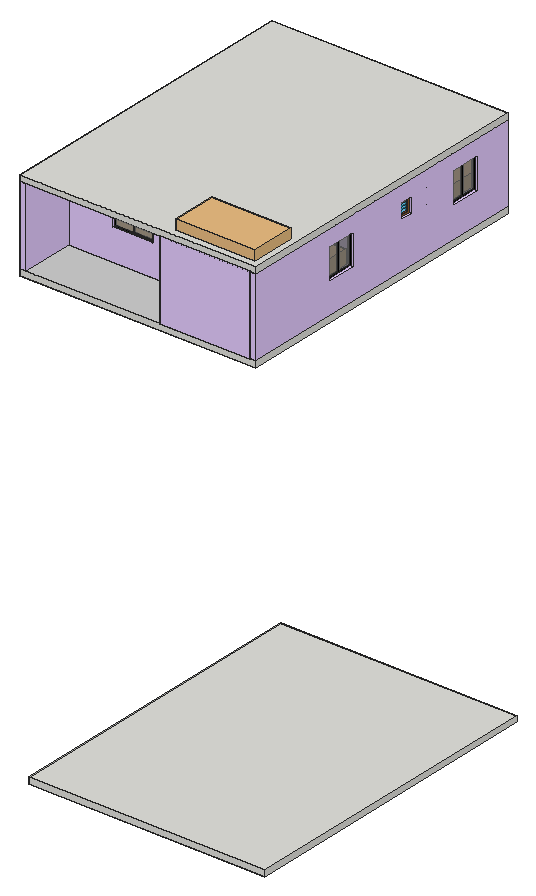
# SketchUp Ruby script. Lengths in inches.
U = 1.inch
M = Sketchup.active_model
def pt(a) = Geom::Point3d.new(a.map { |v| v * U })
def face(e, loops, mat)
  f = e.add_face(loops[0].map { |a| pt(a) })
  loops[1..].each { |l| e.add_face(l.map { |a| pt(a) }).erase! }
  f.material = f.back_material = mat if mat
  f
end
# faces: each face lists its corners as indices into pts; further lists are holes
def faces(e, pts, list, mat = nil) = list.each { |f| face(e, (f[0].is_a?(Array) ? f : [f]).map { |l| l.map { |i| pts[i] } }, mat) }
# xy, xz, yz: faces in a plane at the given z, y or x. An outline is a flat list of corners, or four numbers for a rectangle; further outlines are holes
def ring(l) = l.size == 4 ? [[l[0], l[1]], [l[2], l[1]], [l[2], l[3]], [l[0], l[3]]] : l.each_slice(2).to_a
def flat(e, list, mat, &to3) = list.each { |f| face(e, (f[0].is_a?(Array) ? f : [f]).map { |l| ring(l).map { |u, v| to3.(u, v) } }, mat) }
def xy(e, z, list, mat = nil) = flat(e, list, mat) { |x, y| [x, y, z] }
def xz(e, y, list, mat = nil) = flat(e, list, mat) { |x, z| [x, y, z] }
def yz(e, x, list, mat = nil) = flat(e, list, mat) { |y, z| [x, y, z] }
def lines(e, pts, list) = list.each { |a, b| e.add_line(pt(pts[a]), pt(pts[b])) }
# prism: a flat outline (further loops are holes) pulled along v
def prism(e, loops, v, mat = nil)
  f = face(e, loops, mat); d = Geom::Vector3d.new(v.map { |x| x * U })
  f.pushpull(f.normal.samedirection?(d) ? d.length : -d.length)
end
def box(e, o, s, mat = nil) = prism(e, [[o, [o[0] + s[0], o[1], o[2]], [o[0] + s[0], o[1] + s[1], o[2]], [o[0], o[1] + s[1], o[2]]]], [0, 0, s[2]], mat)
def at(x, y, z, deg = 0) = Geom::Transformation.translation(pt([x, y, z])) * Geom::Transformation.rotation(ORIGIN, Z_AXIS, deg.degrees)
def axes(o, x, y, z) = Geom::Transformation.new([*x, 0, *y, 0, *z, 0, *pt(o).to_a, 1])
def part(name) = M.definitions.add(name)
# library, detail: a bought-in or finely detailed component or shape, given as its bounding box
def library(name, o, s) = part(name).tap { |d| box(d.entities, o, s) }
def detail(e, o, s) = box(e.add_group.entities, o, s)
def put(e, d, t, mat = nil) = e.add_instance(d, t).tap { |i| i.material = mat if mat }
def group(e, t, mat = nil) = e.add_group.tap { |g| g.transformation = t; g.material = mat if mat }.entities
root = M.entities
M.materials.add("[0012_Bisque]").color = [255, 228, 196]
M.materials.add("[Carrera Marble]").color = [207, 207, 207]
M.materials.add("[Color A01]").color = [255, 204, 204]
M.materials.add("[Color B02]").color = [255, 178, 153]
M.materials.add("[Color B07]").color = [153, 38, 0]
M.materials.add("[Color C01]").color = [255, 229, 204]
M.materials.add("[Color C02]").color = [255, 204, 153]
M.materials.add("[Color C07]").color = [153, 76, 0]
M.materials.add("[Color J01]").color = [229, 204, 255]
M.materials.add("[Color K01]").color = [255, 204, 255]
M.materials.add("[Color M02]").color = [198, 198, 198]
M.materials.add("[Color M09]").color = [0, 0, 0]
M.materials.add("[Color_008]").color = [30, 30, 30]
M.materials.add("[Color_009]").color = [0, 0, 0]
M.materials.add("[Metal Corrugated Shiny]").color = [193, 193, 193]
M.materials.add("[Stone Marble]").color = [143, 138, 136]
M.materials.add("[Translucent Glass Gray]").color = [128, 128, 128]
M.materials["[Translucent Glass Gray]"].alpha = 0.5
M.materials.add("[Translucent Glass Tinted]1").color = [7, 201, 240]
M.materials["[Translucent Glass Tinted]1"].alpha = 0.48
M.materials.add("[Translucent_Glass_Gray]").color = [128, 128, 128]
M.materials["[Translucent_Glass_Gray]"].alpha = 0.5
M.materials.add("[Wood Cherry Original]").color = [152, 86, 42]
M.materials.add("[Wood Floor Parquet]").color = [145, 89, 39]
M.materials.add("[Wood Veneer 01]").color = [120, 70, 37]
c1 = library("main+door",[0,-0.79,0],[47.24,7.88,82.68])
c2 = library("Gas cooktop",[0,0,34.52],[24.41,48.07,2.63])
c3 = part("Inclined chimney")
g1 = group(c3.entities,at(1.97,2.08,2.89))
xy(g1,0,[[0,7.9,31.3,13.68]])
xy(g1,11.29,[[0,0,31.3,13.68]])
xz(g1,13.68,[[0,0,31.3,11.29]])
yz(g1,0,[[7.9,0,0,11.29,13.68,11.29,13.68,0]])
yz(g1,31.3,[[7.9,0,13.68,0,13.68,11.29,0,11.29]])
g2 = group(c3.entities,at(0,9.85,0.4))
g3 = group(g2,at(0,0.61,0.43))
prism(g3,[[[35.24,0,0],[35.24,-3.39,4.84],[35.24,-3.58,4.7],[35.24,-0.29,0]]],[-35.24,0,0])
g4 = group(g2,at(0,-3.21,4.99))
prism(g4,[[[35.24,-0.2,-0.12],[35.24,-3.16,5],[0,-3.16,5],[0,-0.2,-0.12]]],[0,0.2,0.12])
g5 = group(g2,at(0,-6.27,10.27))
prism(g5,[[[35.24,-0.19,-0.14],[35.24,-3.58,4.7],[0,-3.58,4.7],[0,-0.19,-0.14]]],[0,0.19,0.14])
g6 = group(g2,at(0,0.61,0.43))
prism(g6,[[[35.24,0,0],[35.24,0.96,0],[35.24,-9.52,14.96],[35.24,-10.16,14.51]]],[-35.24,0,0])
g7 = group(c3.entities,at(10.24,3.95,20.8))
box(g7,[0,0,-6.62],[14.76,11.8125,20.56])
g8 = group(c3.entities,at(0,10.1,0))
prism(g8,[[[35.24,0.46,0],[35.24,1.33,0],[35.24,1.33,0.83],[35.24,1.01,0.83],[35.24,0.37,0.83],[35.24,0,0.83],[35.24,0,0.64]]],[-35.24,0,0])
c4 = part("Inclined+chimney")
put(c4.entities,c3,at(34.17,38.97,0.69))
c5 = library("Component\#33",[0,0,0],[60.64,55.48,158.625])
c6 = library("SKT_Nearly Natural 5' Kentia Palm Silk Tree",[-23.18,-17.61,0],[47.48,43.95,59.125])
c7 = library("Bed",[-100.55,9.74,0],[90.43,103.1,58.68])
c8 = library("2222",[-1.18,-2.36,0],[94.72,146.45,38.04])
c9 = library("CS300DRT",[0,0,0],[27.18,17.85,30.31])
c10 = library("Oval wall hanging",[0,0,0],[26.88,1.18,49.49])
c11 = part("ventilator")
g9 = group(c11.entities,at(0,0,0))
xy(g9,0,[[0,0,24,1],[0,1,24,6.83]],"[Wood Floor Parquet]")
xy(g9,1.75,[[2,0,22,6.83]],"[Wood Floor Parquet]")
xy(g9,21.87,[[2,0,22,6.83]],"[Wood Cherry Original]")
xy(g9,23.62,[[0,0,24,1],[0,1,24,6.83]],"[Wood Floor Parquet]")
xz(g9,0,[[[0,0,24,23.62],[2,1.75,22,21.87]]],"[Wood Floor Parquet]")
xz(g9,6.83,[[[0,0,24,23.62],[2,1.75,22,21.87]]],"[Wood Cherry Original]")
yz(g9,0,[[0,0,1,23.62],[1,0,6.83,23.62]],"[Wood Floor Parquet]")
yz(g9,2,[[0,1.75,6.83,1.75,6.83,7.66,0,3.5],[0,3.5,6.83,7.66,6.83,11.8125,0,7.66],[0,7.66,6.83,11.8125,6.83,15.97,0,11.8125],[0,11.8125,6.83,15.97,6.83,20.12,0,15.97],[0,15.97,6.83,20.12,6.83,21.87,0,21.87]],"[Wood Floor Parquet]")
yz(g9,22,[[0,1.75,0,3.5,6.83,7.66,6.83,1.75],[0,3.5,0,7.66,6.83,11.8125,6.83,7.66],[0,7.66,0,11.8125,6.83,15.97,6.83,11.8125],[0,11.8125,0,15.97,6.83,20.12,6.83,15.97],[0,15.97,0,21.87,6.83,21.87,6.83,20.12]],"[Wood Floor Parquet]")
yz(g9,24,[[0,0,1,23.62],[1,0,6.83,23.62]],"[Wood Floor Parquet]")
p = [[2,0,3.5],[2,6.83,7.66],[22,6.83,7.66],[22,0,3.5],[2,6.83,11.8125],[2,0,7.66],
  [22,0,7.66],[22,6.83,11.8125],[2,0,11.8125],[2,6.83,15.97],[22,6.83,15.97],[22,0,11.8125],
  [2,6.83,20.12],[2,0,15.97],[22,0,15.97],[22,6.83,20.12]]
faces(g9,p,[[0,1,2,3],[4,5,6,7],[8,9,10,11]],"[Translucent Glass Tinted]1")
faces(g9,p,[[12,13,14,15]],"[Translucent Glass Gray]")
c12 = part("Group\#32")
xy(c12.entities,0,[[0,0,82.68,1.18]],"[Color_009]")
xy(c12.entities,1.97,[[1.97,0.98,40.35,1.18],[42.32,0.98,80.71,1.18]])
xy(c12.entities,1.97,[[1.97,0,40.35,0.3],[42.32,0,80.71,0.3]],"[Color_009]")
xy(c12.entities,80.71,[[1.97,0,40.35,0.3],[42.32,0,80.71,0.3],[1.97,0.3,40.35,0.98],[42.32,0.3,80.71,0.98],[1.97,0.98,40.35,1.18],
  [42.32,0.98,80.71,1.18]])
xy(c12.entities,82.68,[[0,0,82.68,1.18]],"[Color_008]")
xz(c12.entities,0,[[[0,0,82.68,82.68],[1.97,1.97,40.35,80.71],[42.32,1.97,80.71,80.71]]],"[Color_009]")
xz(c12.entities,0.3,[[1.97,1.97,40.35,80.71],[42.32,1.97,80.71,80.71]],"[Translucent_Glass_Gray]")
xz(c12.entities,0.98,[[1.97,1.97,40.35,80.71],[42.32,1.97,80.71,80.71]],"[Translucent_Glass_Gray]")
xz(c12.entities,1.18,[[[0,0,82.68,82.68],[1.97,1.97,80.71,80.71]],[40.35,1.97,42.32,80.71]],"[Color_009]")
yz(c12.entities,0,[[0,0,1.18,82.68]],"[Color_009]")
yz(c12.entities,1.97,[[0.98,1.97,1.18,80.71]])
yz(c12.entities,1.97,[[0,1.97,0.3,80.71]],"[Color_009]")
yz(c12.entities,40.35,[[0,1.97,0.3,80.71],[0.98,1.97,1.18,80.71]],"[Color_009]")
yz(c12.entities,42.32,[[0,1.97,0.3,80.71],[0.98,1.97,1.18,80.71]])
yz(c12.entities,80.71,[[0,1.97,0.3,80.71],[0.98,1.97,1.18,80.71]],"[Color_009]")
yz(c12.entities,82.68,[[0,0,1.18,82.68]],"[Color_009]")
c13 = library("Group53\#1",[561.19,10.9375,5.6875],[120.56,68.625,137.75])
c14 = part("Vertical frame member")
xy(c14.entities,-6,[[0,-2,2.13,0]])
xy(c14.entities,78,[[0,-2,2.13,0]])
xz(c14.entities,-2,[[0,-6,2.13,78]],"[Color B07]")
xz(c14.entities,0,[[0,-6,2.13,78]])
yz(c14.entities,0,[[-2,-6,0,78]])
yz(c14.entities,2.13,[[-2,-6,0,78]])
c15 = part("Group\#9")
p = [[2,2,2],[2,2,4],[2,-0.06,4]]
lines(c15.entities,p,[[0,1],[1,2]])
g10 = group(c15.entities,at(0,0,0))
xy(g10,2,[[2,0,8,2]])
xy(g10,4,[[0,0,8,2]])
xz(g10,0,[[0,0,2,0,2,2,8,2,8,4,0,4]])
xz(g10,2,[[0,0,0,4,8,4,8,2,2,2,2,0]])
yz(g10,0,[[0,0,2,4]])
yz(g10,2,[[0,0,2,2]])
yz(g10,8,[[0,2,2,4]])
g11 = group(c15.entities,at(8,0,0))
xy(g11,4,[[0,0,2,2]])
xz(g11,0,[[0,0,2,4]])
xz(g11,2,[[0,0,2,4]])
yz(g11,0,[[0,0,2,4]])
yz(g11,2,[[0,0,2,4]])
c16 = part("Cabinet pull")
p = [[1,1,1],[2,1,1],[2,1,0]]
lines(c16.entities,p,[[0,1],[1,2]])
g12 = group(c16.entities,at(0,8,0),"[Metal Corrugated Shiny]")
xy(g12,0,[[0,0,2,1]])
xy(g12,1,[[0,0,2,1]])
xz(g12,0,[[0,0,2,1]])
xz(g12,1,[[0,0,1,1],[1,0,2,1]])
yz(g12,2,[[0,0,1,1]])
g13 = group(c16.entities,at(0,0,0),"[Metal Corrugated Shiny]")
xy(g13,0,[[0,0,0,1,1,1,1,8,2,8,2,0]])
xy(g13,1,[[0,0,2,0,2,8,1,8,1,1,0,1]])
xz(g13,0,[[0,0,2,1]])
xz(g13,1,[[0,0,1,1]])
xz(g13,8,[[1,0,2,1]])
yz(g13,1,[[1,0,8,1]])
yz(g13,2,[[0,0,8,1]])
c17 = part("Rectangular panel")
box(c17.entities,[0,0,0],[0.4375,33.64,17.64])
c18 = part("Group\#14")
xy(c18.entities,18.12,[[0,0,28.25,0.25]])
xz(c18.entities,0,[[0,0,28.25,18.12]])
yz(c18.entities,0,[[0,0.43,0.25,18.12]])
yz(c18.entities,28.25,[[0,0.43,0.25,17.43],[0,17.43,0.25,18.12]])
xy(root,0,[[228.5,1157.72,238.5,1187.97],[238.5,1157.72,248.5,1187.97],[248.5,1157.72,258.5,1187.97],[258.5,1157.72,268.5,1187.97],[268.5,1157.72,278.5,1187.97],
  [278.5,1157.72,288.5,1187.97],[288.5,1157.72,298.5,1187.97],[298.5,1157.72,308.5,1187.97],[308.5,1157.72,318.5,1187.97],[318.5,1157.72,351,1187.97],
  [318.5,1187.97,351,1199.97],[228.5,1199.97,238.5,1230.22],[238.5,1199.97,248.5,1230.22],[248.5,1199.97,258.5,1230.22],[258.5,1199.97,268.5,1230.22],
  [268.5,1199.97,278.5,1230.22],[278.5,1199.97,288.5,1230.22],[288.5,1199.97,298.5,1230.22],[298.5,1199.97,308.5,1230.22],[308.5,1199.97,318.5,1230.22],
  [318.5,1199.97,351,1230.22]])
p = [[-296.69,1230.22,0],[-295.69,1230.22,0],[-296.69,1235.22,0],[-332.69,1230.22,0],[-332.69,1235.22,0],[-295.69,1266.22,0],
  [-296.69,1266.22,0],[81.8,1619.72,48],[81.8,1619.72,96],[33.8,1619.72,96],[33.8,1619.72,48],[212.75,1235.22,0],
  [9,1235.22,0],[9,1541.6,0],[212.75,1541.6,0],[213.32,1157.72,120],[213.32,1230.22,120]]
lines(root,p,[[0,1],[0,2],[3,4],[5,6],[7,8],[8,9],[9,10],[10,7],[11,12],[12,13],[14,11],[15,16]])
put(root,c1,axes([261.5,1465.22,0],[0,-0.762,0],[0.735,0,0],[0,0,1.016]))
put(root,c2,at(9.27,1518.85,9.47))
put(root,c4,axes([63.73,1499.16,69.82],[0,0.81,0],[-1,0,0],[0,0,0.88]))
put(root,c5,axes([35.81,1464.81,0],[0,0.46858,0],[-0.5529,0,0],[0,0,0.52253]))
put(root,c6,axes([24.22,1605.45,43.99],[0.68,0,0],[0,0.68,0],[0,0,0.5236]))
put(root,c7,axes([226.75,1495.01,0],[0,-1.24,0],[1,0,0],[0,0,1]))
put(root,c7,axes([348.23,1359.9,0],[0,1.24,0],[-1,0,0],[0,0,1]))
put(root,c8,at(29.45,1246.26,0))
put(root,c9,axes([134.5,1569.67,0],[1.5,0,0],[0,1.5,0],[0,0,1.5]))
put(root,c10,axes([162.44,1617.36,58.25],[1,0,0],[0,2,0],[0,0,1]))
put(root,c9,axes([351,1451.89,0],[-1.5,0,0],[0,-1.5,0],[0,0,1.5]))
g14 = group(root,at(0,1148.64,0),"[Color J01]")
xy(g14,0,[[213.32,0,213.32,9.09,351,9.09,351,81.59,208.5,81.59,208.5,86.59,213.5,86.59,213.5,242.59,223.5,242.59,223.5,237.59,218.5,237.59,218.5,86.59,351,86.59,351,186.09,360,186.09,360,0.09,351,0.09,351,0],[0,0.09,0,122.64,9,122.64,9,86.59,136.5,86.59,136.5,81.59,9,81.59,9,0.09],[136.5,81.59,172.5,86.59],[0,122.64,9,239.89],[351,186.09,351,237.59,259.5,237.59,259.5,242.59,261.5,242.59,261.5,280.59,266.5,280.59,266.5,242.59,351,242.59,351,296.33,360,296.33,360,186.09],
  [0,239.89,9,240.09],[0,240.09,0,480.09,33.8,480.09,33.8,471.09,9,471.09,9,314.59,129.5,314.59,129.5,319.59,134.5,319.59,134.5,309.59,9,309.59,9,240.09],[351,296.33,360,324.16],[261.5,316.59,261.5,321.59,259.5,321.59,259.5,326.59,351,326.59,351,422.84,360,422.84,360,324.16,351,324.16,351,321.59,266.5,321.59,266.5,316.59],[213.5,321.59,213.5,471.09,134.5,471.09,134.5,398.59,174.5,398.59,174.5,393.59,134.5,393.59,134.5,355.59,129.5,355.59,129.5,471.09,33.8,471.09,33.8,480.09,260.75,480.09,260.75,471.09,218.5,471.09,218.5,326.59,223.5,326.59,223.5,321.59],
  [211.5,393.59,213.5,398.59],[351,422.84,351,471.09,260.75,471.09,260.75,480.09,360,480.09,360,422.84]])
xy(g14,48,[[76.5,81.59,136.5,86.59],[0,122.64,9,170.84],[351,138.09,360,186.09],[0,239.89,9,288.09],[351,374.84,360,422.84],
  [33.8,471.09,81.8,480.09],[260.75,471.09,308.75,480.09]])
xy(g14,72,[[351,276.16,360,296.33]])
xy(g14,84,[[172.5,81.59,208.5,86.59],[223.5,237.59,259.5,242.59],[261.5,280.59,266.5,316.59],[129.5,319.59,134.5,355.59],[223.5,321.59,259.5,326.59],
  [174.5,393.59,211.5,398.59]])
xy(g14,96,[[76.5,81.59,136.5,86.59],[0,122.64,9,170.84],[351,138.09,360,186.09],[0,239.89,9,288.09],[351,374.84,360,422.84],
  [33.8,471.09,81.8,480.09],[260.75,471.09,308.75,480.09]])
xy(g14,120,[[[213.32,0,351,0,351,0.09,360,0.09,360,480.09,0,480.09,0,0.09,9,0.09,9,81.59,351,81.59,351,9.09,213.32,9.09],[9,86.59,9,309.59,134.5,309.59,134.5,393.59,211.5,393.59,211.5,398.59,134.5,398.59,134.5,471.09,213.5,471.09,213.5,321.59,260.5,321.59,260.5,326.59,218.5,326.59,218.5,471.09,351,471.09,351,326.59,260.5,326.59,260.5,321.59,261.5,321.59,261.5,242.59,213.5,242.59,213.5,86.59],[218.5,86.59,351,237.59],[9,314.59,129.5,471.09],[266.5,242.59,351,321.59]],[211.5,393.59,213.5,398.59]])
xz(g14,0,[[213.32,0,351,120]])
xz(g14,0.09,[[0,0,9,120],[351,0,360,120]])
xz(g14,9.09,[[213.32,0,351,120]])
xz(g14,81.59,[[[9,0,172.5,0,172.5,84,208.5,84,208.5,0,351,0,351,120,9,120],[76.5,48,136.5,96]]])
xz(g14,86.59,[[9,0,9,120,136.5,120,136.5,96,76.5,96,76.5,48,136.5,48,136.5,0],[136.5,0,136.5,120,208.5,120,208.5,84,172.5,84,172.5,0],[208.5,0,213.5,120],[218.5,0,351,120]])
xz(g14,122.64,[[0,48,9,96]])
xz(g14,138.09,[[351,48,360,96]])
xz(g14,170.84,[[0,48,9,96]])
xz(g14,186.09,[[351,48,360,96]])
xz(g14,237.59,[[218.5,0,223.5,0,223.5,84,259.5,84,259.5,0,351,0,351,120,218.5,120]])
xz(g14,242.59,[[213.5,0,213.5,120,259.5,120,259.5,84,223.5,84,223.5,0],[259.5,0,261.5,120],[266.5,0,351,120]])
xz(g14,276.16,[[351,72,360,96]])
xz(g14,280.59,[[261.5,0,266.5,84]])
xz(g14,288.09,[[0,48,9,96]])
xz(g14,309.59,[[9,0,134.5,120]])
xz(g14,314.59,[[9,0,129.5,120]])
xz(g14,316.59,[[261.5,0,266.5,84]])
xz(g14,319.59,[[129.5,0,134.5,84]])
xz(g14,321.59,[[213.5,0,223.5,0,223.5,84,260.5,84,260.5,120,213.5,120],[259.5,0,261.5,0,261.5,120,260.5,120,260.5,84,259.5,84],[266.5,0,351,120]])
xz(g14,326.59,[[218.5,0,218.5,120,260.5,120,260.5,84,223.5,84,223.5,0],[259.5,0,259.5,84,260.5,84,260.5,120,351,120,351,0]])
xz(g14,355.59,[[129.5,0,134.5,84]])
xz(g14,374.84,[[351,48,360,96]])
xz(g14,393.59,[[134.5,0,174.5,0,174.5,84,211.5,84,211.5,120,134.5,120],[211.5,0,213.5,120]])
xz(g14,398.59,[[134.5,0,134.5,120,211.5,120,211.5,84,174.5,84,174.5,0],[211.5,0,213.5,120]])
xz(g14,422.84,[[351,48,360,96]])
xz(g14,471.09,[[[9,0,129.5,120],[33.8,48,81.8,96]],[134.5,0,213.5,120],[[218.5,0,351,120],[260.75,48,308.75,96]]])
xz(g14,480.09,[[0,0,33.8,120],[[33.8,0,33.8,48,81.8,48,81.8,96,33.8,96,33.8,120,360,120,360,0],[260.75,48,308.75,96]]])
yz(g14,0,[[[0.09,0,480.09,120],[122.64,48,170.84,96],[240.09,48,288.09,96]]])
yz(g14,9,[[0.09,0,81.59,120],[[86.59,0,309.59,120],[122.64,48,170.84,96],[240.09,48,288.09,96]],[314.59,0,471.09,120]])
yz(g14,33.8,[[471.09,48,480.09,96]])
yz(g14,76.5,[[81.59,48,86.59,96]])
yz(g14,81.8,[[471.09,48,480.09,96]])
yz(g14,129.5,[[314.59,0,314.59,120,471.09,120,471.09,0,355.59,0,355.59,84,319.59,84,319.59,0]])
yz(g14,134.5,[[309.59,0,319.59,120],[355.59,0,393.59,0,393.59,120,319.59,120,319.59,84,355.59,84],[398.59,0,471.09,120]])
yz(g14,136.5,[[81.59,48,86.59,96]])
yz(g14,172.5,[[81.59,0,86.59,84]])
yz(g14,174.5,[[393.59,0,398.59,84]])
yz(g14,208.5,[[81.59,0,86.59,84]])
yz(g14,211.5,[[393.59,0,398.59,84]])
yz(g14,213.32,[[0,0,9.09,120]])
yz(g14,213.5,[[86.59,0,242.59,120],[321.59,0,393.59,120],[393.59,0,398.59,120],[398.59,0,471.09,120]])
yz(g14,218.5,[[86.59,0,237.59,120],[326.59,0,471.09,120]])
yz(g14,223.5,[[237.59,0,242.59,84],[321.59,0,326.59,84]])
yz(g14,259.5,[[237.59,0,242.59,84],[321.59,0,326.59,84]])
yz(g14,260.75,[[471.09,48,480.09,96]])
yz(g14,261.5,[[242.59,0,242.59,120,321.59,120,321.59,0,316.59,0,316.59,84,280.59,84,280.59,0]])
yz(g14,266.5,[[242.59,0,280.59,0,280.59,84,316.59,84,316.59,0,321.59,0,321.59,120,242.59,120]])
yz(g14,308.75,[[471.09,48,480.09,96]])
yz(g14,351,[[0,0,0.09,120],[9.09,0,81.59,120],[86.59,0,86.59,120,186.09,120,186.09,96,138.09,96,138.09,48,186.09,48,186.09,0],[186.09,0,237.59,120],[[242.59,0,321.59,120],[276.16,72,296.33,96]],
  [321.59,0,324.16,72],[[326.59,0,471.09,120],[374.84,48,422.84,96]]])
yz(g14,360,[[[0.09,0,480.09,120],[138.09,48,186.09,96],[374.84,48,422.84,96],[276.16,72,296.33,96]]])
p = [[360,324.16,72],[351,324.16,72],[360,324.16,96],[351,324.16,96],[351,321.59,96],[351,0.09,0],
  [351,0.46,0]]
lines(g14,p,[[0,1],[2,3],[4,3],[5,6]])
put(g14,c11,axes([355.5,276.16,72],[0,0.84037,0],[-0.35,0,0],[0,0,1.016]))
put(g14,c1,axes([223.5,237.38,0],[0.762,0,0],[0,0.735,0],[0,0,1.016]))
put(g14,c1,axes([129.5,355.59,0],[0,-0.762,0],[0.735,0,0],[0,0,1.016]))
put(g14,c1,axes([223.5,321.59,0],[0.762,0,0],[0,0.735,0],[0,0,1.016]))
put(g14,c1,axes([172.5,81.38,0],[0.762,0,0],[0,0.735,0],[0,0,1.016]))
put(g14,c1,axes([174.5,393.59,0],[0.762,0,0],[0,0.735,0],[0,0,1.016]))
put(g14,c12,axes([3.32,288.09,48],[0,-0.58057,0],[1,0,0],[0,0,0.5852]))
g15 = group(g14,at(33.8,475.59,48))
xy(g15,0,[[0,0,48,1.18]],"[Color_009]")
xy(g15,1.15,[[1.14,0.98,23.43,1.18],[24.57,0.98,46.86,1.18]])
xy(g15,1.15,[[1.14,0,23.43,0.3],[24.57,0,46.86,0.3]],"[Color_009]")
xy(g15,47.23,[[1.14,0,23.43,0.3],[24.57,0,46.86,0.3],[1.14,0.3,23.43,0.98],[24.57,0.3,46.86,0.98],[1.14,0.98,23.43,1.18],
  [24.57,0.98,46.86,1.18]])
xy(g15,48.38,[[0,0,48,1.18]],"[Color_008]")
xz(g15,0,[[[0,0,48,48.38],[1.14,1.15,23.43,47.23],[24.57,1.15,46.86,47.23]]],"[Color_009]")
xz(g15,0.3,[[1.14,1.15,23.43,47.23],[24.57,1.15,46.86,47.23]],"[Translucent_Glass_Gray]")
xz(g15,0.98,[[1.14,1.15,23.43,47.23],[24.57,1.15,46.86,47.23]],"[Translucent_Glass_Gray]")
xz(g15,1.18,[[[0,0,48,48.38],[1.14,1.15,46.86,47.23]],[23.43,1.15,24.57,47.23]],"[Color_009]")
yz(g15,0,[[0,0,1.18,48.38]],"[Color_009]")
yz(g15,1.14,[[0.98,1.15,1.18,47.23]])
yz(g15,1.14,[[0,1.15,0.3,47.23]],"[Color_009]")
yz(g15,23.43,[[0,1.15,0.3,47.23],[0.98,1.15,1.18,47.23]],"[Color_009]")
yz(g15,24.57,[[0,1.15,0.3,47.23],[0.98,1.15,1.18,47.23]])
yz(g15,46.86,[[0,1.15,0.3,47.23],[0.98,1.15,1.18,47.23]],"[Color_009]")
yz(g15,48,[[0,0,1.18,48.38]],"[Color_009]")
put(g14,c12,axes([260.75,475.59,48],[0.58057,0,0],[0,1,0],[0,0,0.5852]))
put(g14,c12,axes([354.32,422.84,48],[0,-0.58057,0],[1,0,0],[0,0,0.5852]))
put(g14,c12,axes([354.32,186.09,48],[0,-0.58057,0],[1,0,0],[0,0,0.5852]))
put(g14,c12,axes([3.32,170.84,48],[0,-0.58057,0],[1,0,0],[0,0,0.5852]))
put(g14,c12,axes([136.5,84.09,48],[-0.72571,0,0],[0,1,0],[0,0,0.58057]))
put(root,c13,at(-332.69,1148.72,0))
g16 = group(root,at(228.5,1157.72,-5.0625))
xy(g16,0,[[10,42.25,20,72.5]])
xy(g16,5.0625,[[0,42.25,10,72.5]])
xy(g16,5.6875,[[20,42.25,30,72.5]])
xy(g16,10.75,[[0,42.25,10,72.5]])
xy(g16,11.375,[[30,42.25,40,72.5]])
xy(g16,16.4375,[[10,42.25,20,72.5]])
xy(g16,17.0625,[[40,42.25,50,72.5]])
xy(g16,22.125,[[20,42.25,30,72.5]])
xy(g16,22.75,[[50,42.25,60,72.5]])
xy(g16,27.8125,[[30,42.25,40,72.5]])
xy(g16,33.5,[[40,42.25,50,72.5]])
xy(g16,34.125,[[70,42.25,80,72.5]])
xy(g16,39.1875,[[50,42.25,60,72.5]])
xy(g16,39.8125,[[80,42.25,90,72.5]])
xy(g16,44.875,[[60,42.25,70,72.5]])
xy(g16,45.5,[[90,42.25,122.5,72.5]])
xy(g16,50.5625,[[70,42.25,80,72.5]])
xy(g16,51.1875,[[90,30.25,122.5,42.25]])
xy(g16,56.25,[[80,42.25,90,72.5]])
xy(g16,56.875,[[90,0,122.5,30.25]])
xy(g16,61.9375,[[90,42.25,122.5,72.5]])
xy(g16,62.5625,[[80,0,90,30.25]])
xy(g16,67.625,[[90,30.25,122.5,42.25]])
xy(g16,68.25,[[70,0,80,30.25]])
xy(g16,73.3125,[[90,0,122.5,30.25]])
xy(g16,73.9375,[[60,0,70,30.25]])
xy(g16,79,[[80,0,90,30.25]])
xy(g16,79.625,[[50,0,60,30.25]])
xy(g16,84.6875,[[70,0,80,30.25]])
xy(g16,85.3125,[[40,0,50,30.25]])
xy(g16,90.375,[[60,0,70,30.25]])
xy(g16,91,[[30,0,40,30.25]])
xy(g16,96.0625,[[50,0,60,30.25]])
xy(g16,96.6875,[[20,0,30,30.25]])
xy(g16,101.75,[[40,0,50,30.25]])
xy(g16,102.375,[[10,0,20,30.25]])
xy(g16,107.4375,[[30,0,40,30.25]])
xy(g16,108.0625,[[0,0,10,30.25]])
xy(g16,113.125,[[20,0,30,30.25]])
xy(g16,118.8125,[[10,0,20,30.25]])
xy(g16,124.5,[[0,0,10,30.25]])
xz(g16,0,[[90,56.875,122.5,56.875,122.5,73.3125,90,73.3125,90,79,80,79,80,84.6875,70,84.6875,70,90.375,60,90.375,60,96.0625,50,96.0625,50,101.75,40,101.75,40,107.4375,30,107.4375,30,113.125,20,113.125,20,118.8125,10,118.8125,10,124.5,0,124.5,0,108.0625,10,108.0625,10,102.375,20,102.375,20,96.6875,30,96.6875,30,91,40,91,40,85.3125,50,85.3125,50,79.625,60,79.625,60,73.9375,70,73.9375,70,68.25,80,68.25,80,62.5625,90,62.5625]])
xz(g16,30.25,[[90,51.1875,122.5,56.875],[80,62.5625,80,68.25,70,68.25,70,73.9375,60,73.9375,60,79.625,50,79.625,50,85.3125,40,85.3125,40,91,30,91,30,96.6875,20,96.6875,20,102.375,10,102.375,10,108.0625,0,108.0625,0,124.5,10,124.5,10,118.8125,20,118.8125,20,113.125,30,113.125,30,107.4375,40,107.4375,40,101.75,50,101.75,50,96.0625,60,96.0625,60,90.375,70,90.375,70,84.6875,80,84.6875,80,79,90,79,90,73.3125,122.5,73.3125,122.5,67.625,90,67.625,90,62.5625]])
xz(g16,42.25,[[10,0,20,0,20,5.6875,30,5.6875,30,11.375,40,11.375,40,17.0625,50,17.0625,50,22.75,60,22.75,60,28.4375,70,34.125,80,34.125,80,39.8125,90,39.8125,90,45.5,122.5,45.5,122.5,51.1875,90,51.1875,90,56.25,80,56.25,80,50.5625,70,50.5625,70,44.875,60,44.875,60,39.1875,50,39.1875,50,33.5,40,33.5,40,27.8125,30,27.8125,30,22.125,20,22.125,20,16.4375,10,16.4375,10,10.75,0,10.75,0,5.0625,10,5.0625],[90,61.9375,122.5,67.625]])
xz(g16,72.5,[[10,0,10,5.0625,0,5.0625,0,10.75,10,10.75,10,16.4375,20,16.4375,20,22.125,30,22.125,30,27.8125,40,27.8125,40,33.5,50,33.5,50,39.1875,60,39.1875,60,44.875,70,44.875,70,50.5625,80,50.5625,80,56.25,90,56.25,90,61.9375,122.5,61.9375,122.5,45.5,90,45.5,90,39.8125,80,39.8125,80,34.125,70,34.125,60,28.4375,60,22.75,50,22.75,50,17.0625,40,17.0625,40,11.375,30,11.375,30,5.6875,20,5.6875,20,0]])
yz(g16,0,[[42.25,5.0625,72.5,10.75],[0,108.0625,30.25,124.5]])
yz(g16,10,[[42.25,0,72.5,5.0625],[42.25,10.75,72.5,16.4375],[0,102.375,30.25,108.0625],[0,118.8125,30.25,124.5]])
yz(g16,20,[[42.25,0,72.5,5.6875],[42.25,16.4375,72.5,22.125],[0,96.6875,30.25,102.375],[0,113.125,30.25,118.8125]])
yz(g16,30,[[42.25,5.6875,72.5,11.375],[42.25,22.125,72.5,27.8125],[0,91,30.25,96.6875],[0,107.4375,30.25,113.125]])
yz(g16,40,[[42.25,11.375,72.5,17.0625],[42.25,27.8125,72.5,33.5],[0,85.3125,30.25,91],[0,101.75,30.25,107.4375]])
yz(g16,50,[[42.25,17.0625,72.5,22.75],[42.25,33.5,72.5,39.1875],[0,79.625,30.25,85.3125],[0,96.0625,30.25,101.75]])
yz(g16,60,[[42.25,22.75,72.5,28.4375],[42.25,39.1875,72.5,44.875],[0,73.9375,30.25,79.625],[0,90.375,30.25,96.0625]])
yz(g16,70,[[42.25,44.875,72.5,50.5625],[0,68.25,30.25,73.9375],[0,84.6875,30.25,90.375]])
yz(g16,80,[[42.25,34.125,72.5,39.8125],[42.25,50.5625,72.5,56.25],[0,62.5625,30.25,68.25],[0,79,30.25,84.6875]])
yz(g16,90,[[42.25,39.8125,72.5,45.5],[30.25,51.1875,30.25,56.875,0,56.875,0,62.5625,30.25,62.5625,30.25,67.625,42.25,67.625,42.25,61.9375,72.5,61.9375,72.5,56.25,42.25,56.25,42.25,51.1875],[0,73.3125,30.25,79]])
yz(g16,122.5,[[42.25,45.5,72.5,45.5,72.5,61.9375,42.25,61.9375,42.25,67.625,30.25,67.625,30.25,73.3125,0,73.3125,0,56.875,30.25,56.875,30.25,51.1875,42.25,51.1875]])
p = [[70,42.25,34.125],[60,42.25,28.4375],[60,72.5,28.4375],[70,72.5,34.125],[0,0,124.5],[0,0,130.1875],
  [0,30.25,130.1875],[0,30.25,124.5]]
faces(g16,p,[[0,1,2,3]])
lines(g16,p,[[4,5],[6,7]])
g17 = group(root,at(0,1148.72,-9))
xy(g17,0,[[0,0,360,480]])
xy(g17,9,[[0,0,360,480]],"[Carrera Marble]")
xz(g17,0,[[0,0,360,9]])
xz(g17,480,[[0,0,360,9]])
yz(g17,0,[[0,0,480,9]])
yz(g17,360,[[0,0,480,9]])
g18 = group(root,at(9.5,1458.22,0))
xy(g18,0,[[0,-18,125,0]])
xy(g18,6,[[0,-20,125,-18]])
xy(g18,7.52,[[74.02,-21,97.98,-20],[98.02,-21,123.48,-20]])
xy(g18,7.53,[[26.03,-21,49.97,-20],[50.03,-21,73.97,-20]])
xy(g18,7.54,[[1.54,-21,25.96,-20]])
xy(g18,8.53,[[51.03,-21,72.97,0]])
xy(g18,14,[[51.03,-21,72.97,0]])
xy(g18,16,[[51.03,-21,72.97,0]])
xy(g18,21.47,[[51.03,-21,72.97,0]])
xy(g18,22.46,[[1.54,-21,25.96,-20]])
xy(g18,22.47,[[26.03,-21,49.97,-20],[50.03,-21,73.97,-20]])
xy(g18,22.48,[[0,-26,74.02,-20],[74.02,-26,97.98,-21],[97.98,-26,98.02,-20],[98.02,-26,123.48,-21],[123.48,-26,125,-20],
  [74.02,-21,97.98,-20],[98.02,-21,123.48,-20]])
xy(g18,24,[[0,-26,125,0]],"[Color B02]")
xy(g18,54,[[123.81,-19.96,93.67,-17.96,94.87,0,125,-2],[2.13,-18.25,31.01,0]])
xy(g18,54.24,[[32.68,-2,91.87,0]])
xy(g18,56.14,[[2.13,-18.25,31.01,0]],"[0012_Bisque]")
xy(g18,56.62,[[123.81,-19.96,125,-2,94.87,0,93.67,-17.96]],"[0012_Bisque]")
xy(g18,61.92,[[39.74,-4,84.49,-2]],"[Color M09]")
xy(g18,71.875,[[123.81,-19.96,93.67,-17.96,94.87,0,125,-2]])
xy(g18,72,[[2.13,-18.18,31.01,0]])
xy(g18,74.2,[[2.13,-18.18,31.01,0]],"[0012_Bisque]")
xy(g18,74.5,[[123.81,-19.96,125,-2,94.87,0,93.67,-17.96]],"[0012_Bisque]")
xy(g18,83.11,[[39.74,-4,84.49,-2]],"[Color M09]")
xy(g18,88.74,[[32.68,-2,91.87,0]])
xy(g18,89.9375,[[123.81,-19.96,93.67,-17.96,94.87,0,125,-2]])
xy(g18,90,[[2.13,-18.17,31.01,0]])
xy(g18,91.75,[[2.13,-18.17,31.01,0]],"[0012_Bisque]")
xy(g18,92.56,[[123.81,-19.96,125,-2,94.87,0,93.67,-17.96]],"[0012_Bisque]")
xy(g18,108,[[0,-18,2.13,0]])
xy(g18,108,[[2.13,-18,125,0]],"[Color K01]")
xy(g18,114,[[0,-18,125,0]],"[Color B07]")
xz(g18,-26,[[0,22.48,125,24]],"[Color C01]")
xz(g18,-21,[[74.02,7.52,97.98,22.48],[98.02,7.52,123.48,22.48],[26.03,7.53,49.97,22.47],[[50.03,7.53,73.97,15],[51.03,8.53,72.97,14]],[1.54,7.54,25.96,22.46],
  [[50.03,15,73.97,22.47],[51.03,16,72.97,21.47]]],"[Color C07]")
xz(g18,-20,[[0,6,125,6,125,22.48,123.48,22.48,123.48,7.52,98.02,7.52,98.02,22,97.98,22,97.98,7.52,74.02,7.52,74.02,8,73.97,8,73.97,7.53,50.03,7.53,50.03,8,49.97,8,49.97,7.53,26.03,7.53,26.03,22.47,49.97,22.47,49.97,22,50.03,22,50.03,22.47,73.97,22.47,73.97,22,74.02,22,74.02,22.48,0,22.48,0,22.46,25.96,22.46,25.96,7.54,1.54,7.54,1.54,22.46,0,22.46],[74.02,7.52,97.98,22.48],[98.02,7.52,123.48,22.48],[49.97,8,50.03,22],[73.97,8,74.02,22],
  [97.98,22,98.02,22.48]])
xz(g18,-18.25,[[2.13,54,31.01,56.14]],"[Color B07]")
xz(g18,-18.18,[[2.13,72,31.01,74.2]],"[Color B07]")
xz(g18,-18.17,[[2.13,90,31.01,91.75]],"[Color B07]")
xz(g18,-18,[[0,108,125,114]],"[Color B07]")
xz(g18,-18,[[0,0,125,6]],"[Color C07]")
xz(g18,-4,[[39.74,61.92,84.49,83.11]],"[Color M09]")
xz(g18,-2,[[[32.68,54.24,91.87,88.74],[39.74,61.92,84.49,83.11]]],"[Color A01]")
xz(g18,0,[[25.5,8,26.5,22],[49.5,8,50.5,22],[73.5,8,74.5,22],[97.5,8,98.5,22],[51.03,8.53,72.97,14],
  [51.03,16,72.97,21.47],[0,108,125,114]])
xz(g18,0,[[[2.13,30,125,30,125,108,2.13,108,2.13,91.75,31.01,91.75,31.01,90,2.13,90,2.13,74.2,31.01,74.2,31.01,72,2.13,72,2.13,56.14,31.01,56.14,31.01,54,2.13,54],[32.68,54.24,91.87,88.74]]],"[Color A01]")
xz(g18,0,[[0,24,125,30]],"[Color C02]")
yz(g18,0,[[-18,0,0,6],[-20,6,0,22.48],[-26,22.48,0,24],[-18,108,0,114]])
yz(g18,1.54,[[-21,7.54,-20,22.46]])
yz(g18,2.13,[[-18.25,54,0,56.14],[-18.18,72,0,74.2],[-18.17,90,0,91.75]])
yz(g18,25.96,[[-21,7.54,-20,22.46]])
yz(g18,26.03,[[-21,7.53,-20,22.47]])
yz(g18,31.01,[[-18.25,54,0,56.14],[-18.18,72,0,74.2],[-18.17,90,0,91.75]],"[0012_Bisque]")
yz(g18,32.68,[[-2,54.24,0,88.74]])
yz(g18,39.74,[[-4,61.92,-2,83.11]],"[Color M09]")
yz(g18,49.97,[[-21,7.53,-20,8],[-21,8,-20,22],[-21,22,-20,22.47]])
yz(g18,50.03,[[-21,7.53,-20,8],[-21,8,-20,22],[-21,22,-20,22.47]])
yz(g18,51.03,[[-21,8.53,0,14],[-21,16,0,21.47]])
yz(g18,72.97,[[-21,8.53,0,14],[-21,16,0,21.47]])
yz(g18,73.97,[[-21,7.53,-20,8],[-21,8,-20,22],[-21,22,-20,22.47]])
yz(g18,74.02,[[-21,7.52,-20,8],[-21,8,-20,22],[-21,22,-20,22.48]])
yz(g18,84.49,[[-4,61.92,-2,83.11]],"[Color M09]")
yz(g18,91.87,[[-2,54.24,0,88.74]])
yz(g18,97.98,[[-21,7.52,-20,22],[-21,22,-20,22.48]])
yz(g18,98.02,[[-21,7.52,-20,22],[-21,22,-20,22.48]])
yz(g18,123.48,[[-21,7.52,-20,22.48]])
yz(g18,125,[[-18,0,0,6],[-20,6,0,22.48],[-26,22.48,0,24],[-18,108,0,114]])
p = [[93.67,-17.96,56.62],[93.67,-17.96,54],[123.81,-19.96,54],[123.81,-19.96,56.62],[125,-2,54],[125,-2,56.62],
  [94.87,0,56.62],[94.87,0,54],[93.67,-17.96,74.5],[93.67,-17.96,71.875],[123.81,-19.96,71.875],[123.81,-19.96,74.5],
  [125,-2,71.875],[125,-2,74.5],[94.87,0,74.5],[94.87,0,71.875],[93.67,-17.96,92.56],[93.67,-17.96,89.9375],
  [123.81,-19.96,89.9375],[123.81,-19.96,92.56],[125,-2,89.9375],[125,-2,92.56],[94.87,0,92.56],[94.87,0,89.9375],
  [25.5,0,8],[25.5,-20,8],[26.5,0,22],[26.5,-20,22],[50.5,0,22],[50.5,-20,22],
  [74.5,0,22],[74.5,-20,22],[98.5,0,22],[98.5,-20,22],[97.5,0,8],[97.5,-20,8],
  [49.5,0,8],[49.5,-20,8],[25.5,0,22],[25.5,-20,22],[26.5,0,8],[26.5,-20,8],
  [49.5,0,22],[49.5,-20,22],[50.5,0,8],[50.5,-20,8],[73.5,0,22],[73.5,-20,22],
  [97.5,0,22],[97.5,-20,22],[98.5,0,8],[98.5,-20,8],[7.77,-23,18.09],[7.77,-25,18.09],
  [7.77,-25,16.09],[73.97,-21,15],[74.02,-21,15]]
faces(g18,p,[[0,1,2,3],[8,9,10,11],[16,17,18,19]],"[Color B07]")
faces(g18,p,[[4,5,3,2],[6,7,1,0],[7,6,5,4],[12,13,11,10],[14,15,9,8],[15,14,13,12],[20,21,19,18],[22,23,17,16],
  [23,22,21,20]])
lines(g18,p,[[24,25],[26,27],[28,29],[30,31],[32,33],[34,35],[36,37],[38,39],[40,41],[42,43],[44,45],[46,47],
  [48,49],[50,51],[52,53],[53,54],[55,56]])
put(g18,c14,at(0,0,30))
put(g18,c14,at(4,0,30))
put(g18,c14,at(8,0,30))
put(g18,c14,at(12,0,30))
put(g18,c14,at(16,0,30))
put(g18,c14,at(20,0,30))
put(g18,c14,at(24,0,30))
put(g18,c14,at(28,0,30))
put(g18,c14,at(122.87,0,30))
put(g18,c14,at(118.87,0,30))
put(g18,c14,at(114.87,0,30))
put(g18,c14,at(110.87,0,30))
put(g18,c14,at(106.87,0,30))
put(g18,c14,at(102.87,0,30))
put(g18,c14,at(98.87,0,30))
put(g18,c14,at(94.87,0,30))
put(g18,c15,axes([8.4,-21,16.09],[1,0,0],[0,0,1],[0,-1,0]))
put(g18,c15,axes([33.77,-21,16.09],[1,0,0],[0,0,1],[0,-1,0]))
put(g18,c15,axes([81.27,-21,16.09],[1,0,0],[0,0,1],[0,-1,0]))
put(g18,c15,axes([105.52,-21,16.09],[1,0,0],[0,0,1],[0,-1,0]))
g19 = group(root,at(9,1463.22,0),"[Carrera Marble]")
xy(g19,42,[[26,29.83,0,30,0.82,156.5,0.82,130.25,26.65,130.25],[0.82,130.25,26.65,130.25,26.82,156.33,0.82,156.5],[26.65,130.25,120.5,130.25,120.5,156.5,0.82,156.5,26.82,156.33]])
xy(g19,43.99,[[26,29.83,0,30,0.82,156.5,120.5,156.5,120.5,130.25,26.65,130.25]],"[Stone Marble]")
xy(g19,78,[[0,30,12,61.625],[0,61.625,12,62.625],[0,92.25,12,93.25],[0,93.25,12,124.875],[0,124.875,12,156.5]])
xy(g19,79,[[0,94.25,12,123.875],[0,125.875,12,155.25]],"[Wood Veneer 01]")
xy(g19,101,[[0,62.625,12,82],[0,82,12,92.25]])
xy(g19,101,[[0,94.25,12,108],[0,108,12,123.875],[0,125.875,12,134],[0,134,12,155.25]],"[Wood Veneer 01]")
xy(g19,102,[[0,0,12,30],[12,144.5,33.6,156.5],[33.6,144.5,38,156.5],[38,144.5,55.2,156.5],[55.2,144.5,76.8,156.5],
  [76.8,144.5,98.4,156.5],[98.4,144.5,120,156.5]])
xy(g19,102.96,[[77.76,143.5,98.07,144.5]])
xy(g19,102.98,[[12.98,143.5,33.12,144.5],[34.08,143.5,38,144.5],[38,143.5,54.47,144.5],[56.18,143.5,75.94,144.5],[98.94,143.5,119.52,144.5]])
xy(g19,103,[[12,1,13,29],[12,31,13,55.5],[12,56.5,13,61.625],[12,61.625,13,81.5],[12,82.5,13,93.25],
  [12,93.25,13,107.5],[12,108.5,13,124.875],[12,124.875,13,133.5]])
xy(g19,119,[[12,1,13,29],[12,31,13,55.5],[12,56.5,13,81.5],[12,82.5,13,107.5],[12,108.5,13,133.5]])
xy(g19,119.02,[[12.98,143.5,33.12,144.5],[34.08,143.5,54.47,144.5],[56.18,143.5,75.94,144.5],[98.94,143.5,119.52,144.5]])
xy(g19,119.04,[[77.76,143.5,98.07,144.5]])
xy(g19,120,[[0,0,12,30],[0,30,12,56],[0,56,12,82],[0,82,12,108],[0,108,12,134],
  [0,134,12,156.5],[12,144.5,33.6,156.5],[33.6,144.5,55.2,156.5],[55.2,144.5,76.8,156.5],[76.8,144.5,98.4,156.5],
  [98.4,144.5,120,156.5]])
xz(g19,0,[[0,0,120.5,0,120.5,120,12,120,12,102,0,102]])
xz(g19,1,[[12,103,13,119]])
xz(g19,29,[[12,103,13,119]])
xz(g19,30,[[0,78,12,102]])
xz(g19,31,[[12,103,13,119]])
xz(g19,55.5,[[12,103,13,119]])
xz(g19,56.5,[[12,103,13,119]])
xz(g19,62.625,[[0,78,12,79],[0,79,12,101]])
xz(g19,81.5,[[12,103,13,119]])
xz(g19,82.5,[[12,103,13,119]])
xz(g19,92.25,[[0,78,12,79],[0,79,12,101]])
xz(g19,94.25,[[0,79,12,101]],"[Wood Veneer 01]")
xz(g19,107.5,[[12,103,13,119]])
xz(g19,108.5,[[12,103,13,119]])
xz(g19,123.875,[[0,79,12,101]],"[Wood Veneer 01]")
xz(g19,125.875,[[0,79,12,101]],"[Wood Veneer 01]")
xz(g19,130.25,[[26.65,42,120.5,43.99]],"[Stone Marble]")
xz(g19,133.5,[[12,103,13,119]])
xz(g19,143.5,[[77.76,102.96,98.07,119.04],[12.98,102.98,33.12,119.02],[34.08,102.98,54.47,119.02],[56.18,102.98,75.94,119.02],[98.94,102.98,119.52,119.02]],"[Color A01]")
xz(g19,144.5,[[[12,102,33.6,120],[12.98,102.98,33.12,119.02]],[[33.6,102,55.2,120],[34.08,102.98,54.47,119.02]],[[55.2,102,76.8,120],[56.18,102.98,75.94,119.02]],[[76.8,102,98.4,120],[77.76,102.96,98.07,119.04]],[[98.4,102,120,120],[98.94,102.98,119.52,119.02]]])
xz(g19,155.25,[[0,79,12,101]],"[Wood Veneer 01]")
xz(g19,156.5,[[[0,0,0,78,12,78,12,102,120.5,102,120.5,43.99,0.82,43.99,0.82,42,120.5,42,120.5,0],[24.8,48,72.8,96]],[120,102,120.5,120]])
yz(g19,0,[[0,0,0,102,30,102,30,78,62.625,78,62.625,101,92.25,101,92.25,78,156.5,78,156.5,0]])
yz(g19,0,[[94.25,79,123.875,101],[125.875,79,155.25,101]],"[Wood Veneer 01]")
yz(g19,0.82,[[130.25,42,156.5,43.99]])
yz(g19,12,[[[30,78,61.625,102],[31,79,60.625,101]],[61.625,78,61.625,102,93.25,102,93.25,78,92.25,78,92.25,101,62.625,101,62.625,78],[[93.25,78,124.875,102],[94.25,79,123.875,101]],[[124.875,78,156.5,102],[125.875,79,155.25,101]],[[0,102,30,120],[1,103,29,119]],
  [[30,102,56,120],[31,103,55.5,119]],[[56,102,82,120],[56.5,103,81.5,119]],[[82,102,108,120],[82.5,103,107.5,119]],[[108,102,134,120],[108.5,103,133.5,119]],[134,102,144.5,120]])
yz(g19,12,[[31,79,60.625,101]],"[Color A01]")
yz(g19,12.98,[[143.5,102.98,144.5,119.02]])
yz(g19,13,[[1,103,29,119],[31,103,55.5,119],[56.5,103,81.5,119],[82.5,103,107.5,119],[108.5,103,133.5,119]],"[Color A01]")
yz(g19,33.12,[[143.5,102.98,144.5,119.02]])
yz(g19,34.08,[[143.5,102.98,144.5,119.02]])
yz(g19,54.47,[[143.5,102.98,144.5,119.02]])
yz(g19,56.18,[[143.5,102.98,144.5,119.02]])
yz(g19,75.94,[[143.5,102.98,144.5,119.02]])
yz(g19,77.76,[[143.5,102.96,144.5,119.04]])
yz(g19,98.07,[[143.5,102.96,144.5,119.04]])
yz(g19,98.94,[[143.5,102.98,144.5,119.02]])
yz(g19,119.52,[[143.5,102.98,144.5,119.02]])
yz(g19,120,[[144.5,102,156.5,120]])
yz(g19,120.5,[[130.25,42,156.5,43.99]])
p = [[0,30,43.99],[0,30,42],[26,29.83,42],[26,29.83,43.99],[26.65,130.25,42],[26.65,130.25,43.99],
  [0.82,156.5,43.99],[0.82,156.5,42],[26.82,156.33,43.99],[26.82,156.33,42],[0,30,78],[37,156.5,101],
  [33.6,156.5,101]]
faces(g19,p,[[0,1,2,3],[1,0,6,7],[7,6,8,9]])
faces(g19,p,[[2,4,5,3]],"[Stone Marble]")
lines(g19,p,[[0,10],[11,12]])
put(g19,c16,at(24.4375,110.91,17.12))
put(g19,c16,at(24.4375,42.78,17.12))
put(g19,c16,at(24.4375,110.91,36))
put(g19,c16,at(24.4375,77.16,36))
put(g19,c16,at(24.4375,77.03,17.12))
put(g19,c16,at(24.4375,42.78,36.43))
put(g19,c16,at(36.56,132.25,35.44,-90))
put(g19,c16,at(70.87,132.25,35.44,-90))
put(g19,c16,at(102.31,132.25,35.44,-90))
put(g19,c16,at(70.93,132.25,17.63,-90))
put(g19,c16,at(34.56,132.25,17.63,-90))
put(g19,c16,at(103.37,132.25,17.63,-90))
g20 = group(g19,at(0,0,0),"[Color M02]")
xy(g20,0,[[0,30,26,130.5],[0,130.5,120.5,156.5]])
xy(g20,6,[[24,30,26,64],[24,64,26,98],[24,98,26,130.5],[24,130.5,120.5,132.5]])
xy(g20,7,[[1,31,24,63.5],[1,64.5,24,97.5],[1,98.5,24,131.5],[25,132.5,57.5,155.5],[58.5,132.5,91.5,155.5],
  [92.5,132.5,119.5,155.5]])
xy(g20,23.5,[[1,31,24,63.5],[1,64.5,24,97.5],[1,98.5,24,131.5],[25,132.5,57.5,155.5],[58.5,132.5,91.5,155.5],
  [92.5,132.5,119.5,155.5]])
xy(g20,23.57,[[92,132.25,120.25,132.5]])
xy(g20,24,[[58.5,132.5,91.5,155.5]])
xy(g20,24.18,[[24,30.18,25,63.82]])
xy(g20,24.5,[[1,64.5,24,97.5],[1,98.5,24,131.5]])
xy(g20,41,[[1,64.5,24,97.5],[1,98.5,24,131.5],[58.5,132.5,91.5,155.5]])
xy(g20,42,[[0,30,24,132.5],[0,132.5,24,156.5],[24,132.5,120.5,156.5]])
xz(g20,30,[[0,0,0,42,24,42,24,6,26,6,26,0]])
xz(g20,31,[[1,7,24,23.5]])
xz(g20,63.5,[[1,7,24,23.5]])
xz(g20,64.5,[[1,7,24,23.5],[1,24.5,24,41]])
xz(g20,97.5,[[1,7,24,23.5],[1,24.5,24,41]])
xz(g20,98.5,[[1,7,24,23.5],[1,24.5,24,41]])
xz(g20,130.5,[[26,0,120.5,6]])
xz(g20,131.5,[[1,7,24,23.5],[1,24.5,24,41]])
xz(g20,132.5,[[24,6,120.5,7],[24,7,25,23.5],[57.5,7,58.5,23.5],[91.5,7,92.5,23.5],[119.5,7,120.5,23.5],
  [24,23.5,24,24,24.56,24,24.56,23.57,57.93,23.57,57.93,24,92,24,92,23.57,120.25,23.57,120.25,24,120.5,24,120.5,23.5],[24,24,24,42,120.5,42,120.5,41,120.25,41,120.25,41.69,92,41.69,92,24,91.5,24,91.5,41,57.93,41,57.93,41.82,24.56,41.82,24.56,24],[57.93,24,58.5,41],[120.25,24,120.5,41]])
xz(g20,155.5,[[25,7,57.5,23.5],[58.5,7,91.5,23.5],[92.5,7,119.5,23.5],[25,24,57.5,41],[58.5,24,91.5,41],
  [92.5,24,119.5,41]])
xz(g20,156.5,[[0,0,24,42],[24,0,120.5,42]])
yz(g20,0,[[30,0,132.5,42],[132.5,0,156.5,42]])
yz(g20,1,[[31,7,63.5,23.5],[64.5,7,97.5,23.5],[98.5,7,131.5,23.5],[31,24.5,63.5,41],[64.5,24.5,97.5,41],
  [98.5,24.5,131.5,41]])
yz(g20,24,[[[30,6,64,24],[31,7,63.5,23.5]],[[64,6,98,24],[64.5,7,97.5,23.5]],[[98,6,132.5,24],[98.5,7,131.5,23.5]],[[30,24,64,42],[30.18,24.18,63.82,41.82]],[[64,24,98,42],[64.5,24.5,97.5,41]],
  [[98,24,132.5,42],[98.5,24.5,131.5,41]]])
yz(g20,24.56,[[132.25,23.57,132.5,24],[132.25,24,132.5,41.82]])
yz(g20,25,[[132.5,7,155.5,23.5]])
yz(g20,26,[[30,0,130.5,6]])
yz(g20,57.5,[[132.5,7,155.5,23.5]])
yz(g20,57.93,[[132.25,23.57,132.5,24]])
yz(g20,58.5,[[132.5,7,155.5,23.5],[132.5,24,155.5,41]])
yz(g20,91.5,[[132.5,7,155.5,23.5],[132.5,24,155.5,41]])
yz(g20,92,[[132.25,23.57,132.5,24]])
yz(g20,92.5,[[132.5,7,155.5,23.5]])
yz(g20,119.5,[[132.5,7,155.5,23.5]])
yz(g20,120.25,[[132.25,23.57,132.5,24]])
yz(g20,120.5,[[130.5,0,130.5,6,132.5,6,132.5,42,156.5,42,156.5,0]])
p = [[120.5,0,0],[0,0,0],[24,31,41],[1,31,41],[24,31,24.5],[1,31,24.5],
  [24,63.5,41],[1,63.5,41],[24,63.5,24.5],[1,63.5,24.5],[57.5,132.5,41],[57.93,132.5,41],
  [119.5,132.5,41],[120.25,132.5,41],[57.5,155.5,41],[25,132.5,41],[25,155.5,41],[25,132.5,24],
  [25,155.5,24],[119.5,155.5,41],[92.5,132.5,41],[92.5,155.5,41],[119.5,132.5,24],[119.5,155.5,24],
  [92.5,132.5,24],[92.5,155.5,24],[24.56,132.5,24],[92,132.5,24],[0,30,0],[120.5,130.5,0]]
lines(g20,p,[[0,1],[2,3],[4,5],[6,7],[8,9],[10,11],[12,13],[10,14],[15,16],[17,18],[12,19],[20,21],
  [22,23],[24,25],[26,17],[27,24],[1,28],[29,0]])
put(g20,c17,at(24,30.18,24.18),"[Wood Cherry Original]")
put(g20,c17,at(24,64.18,24.18),"[Wood Cherry Original]")
put(g20,c17,at(24,98.18,24.18),"[Wood Cherry Original]")
put(g20,c17,at(24,98.18,6.18),"[Wood Cherry Original]")
put(g20,c17,at(24,64.24,6.18),"[Wood Cherry Original]")
put(g20,c17,at(24,30.18,6.18),"[Wood Cherry Original]")
g21 = group(g20,at(58.25,132.25,23.57),"[Wood Cherry Original]")
xy(g21,0,[[0,0,33.375,0.25]])
xy(g21,18.25,[[0,0,33.375,0.25]])
xz(g21,0,[[0,0,33.375,18.25]])
yz(g21,33.375,[[0,0,0.25,17.43],[0,17.43,0.25,18.25]])
g22 = group(g20,at(24.56,132.25,23.57),"[Wood Cherry Original]")
xy(g22,18.25,[[0,0,33.375,0.25]])
xz(g22,0,[[0,0,33.375,18.25]])
yz(g22,33.375,[[0,0,0.25,0.43],[0,0.43,0.25,17.43],[0,17.43,0.25,18.25]])
g23 = group(g20,at(24.56,132.25,5.26),"[Wood Cherry Original]")
xy(g23,0,[[0,0,33.375,0.25]])
xy(g23,0.61,[[0,0,33.375,0.25]])
xy(g23,18.25,[[0,0,33.375,0.25]])
xz(g23,0,[[0,0.61,33.375,18.25]])
xz(g23,0.25,[[0,0,33.375,0.61]])
yz(g23,0,[[0,0,0.25,0.61]])
yz(g23,33.375,[[0,0,0.25,0.43],[0,0.43,0.25,0.61],[0,0.61,0.25,17.43],[0,17.43,0.25,18.25]])
g24 = group(g20,at(58.25,132.25,5.25),"[Wood Cherry Original]")
xy(g24,0,[[0,0,33.375,0.25]])
xy(g24,18.25,[[0,0,33.375,0.25]])
xz(g24,0,[[0,0,33.375,18.25]])
yz(g24,33.375,[[0,0.43,0.25,17.43],[0,17.43,0.25,18.25]])
put(g20,c18,at(92,132.25,23.57),"[Wood Cherry Original]")
put(g20,c18,at(92,132.25,5.38),"[Wood Cherry Original]")
g25 = group(root,at(0,1148.72,120))
box(g25,[0,0,0],[360,480,9])
g26 = group(root,at(932.35,0,127.53))
box(g26,[0,0,0],[360,480,9])
